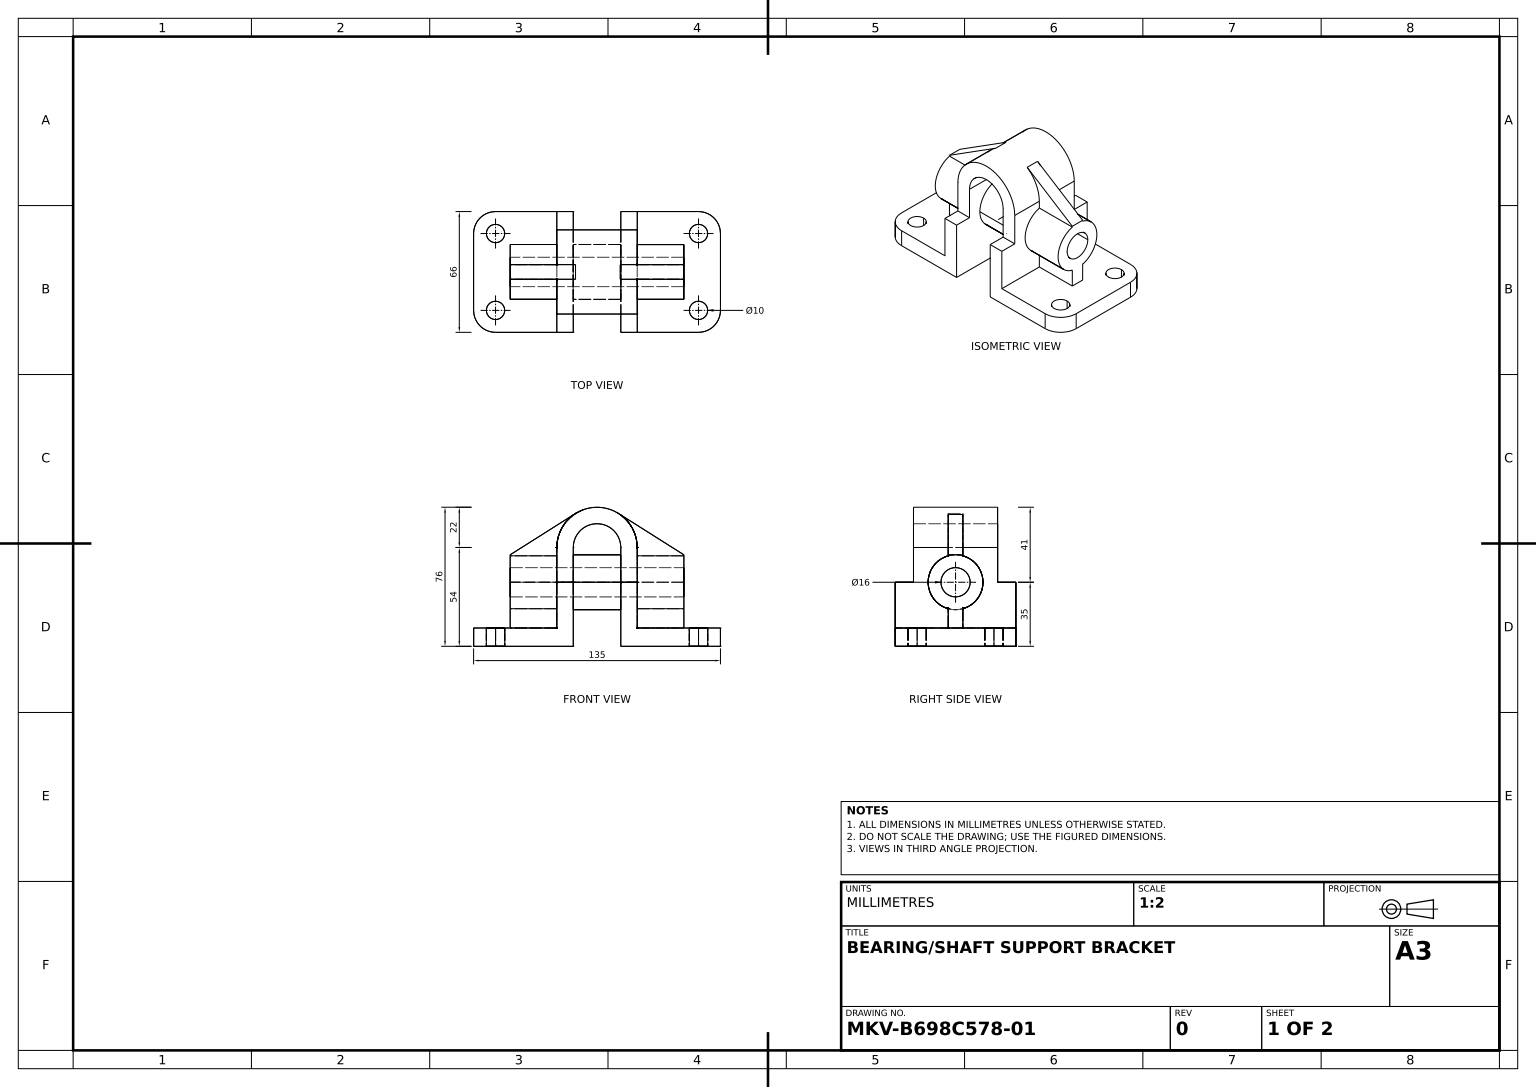
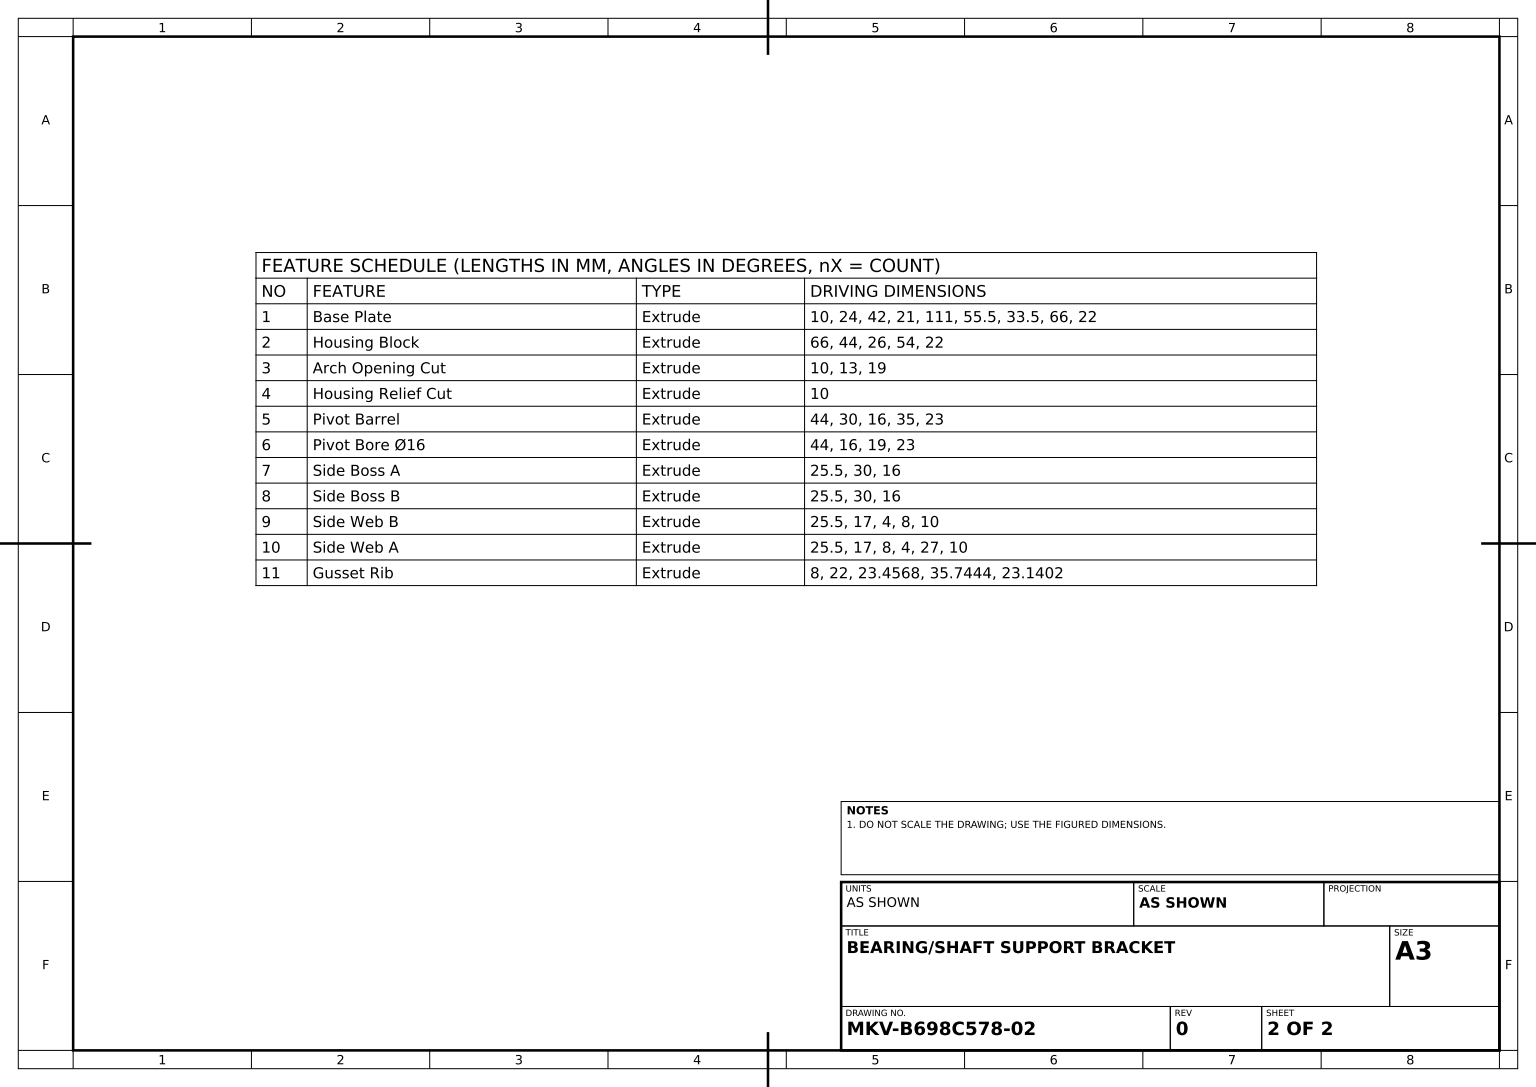
solid
v1 (13,35,15)
v2 (-13,35,15)
e1 v1 v2 LINE
v3 (-13,35,-15)
e2 v2 v3 CIRCLE(AX(P(-13,35,0),D(1,0,0),D(0,0,-1)),15)
v4 (13,35,-15)
e3 v4 v3 LINE
e4 v4 v1 CIRCLE(AX(P(13,35,0),D(-1,0,0),D(0,0,1)),15)
face CYL(AX(P(22,35,0),D(-1,0,0),D(0,0,1)),15) [e1 e2 -e3 e4]
v5 (-67.5,10,21)
v6 (-55.5,10,33)
e5 v5 v6 CIRCLE(AX(P(-55.5,10,21),D(0,1,0),D(0,0,1)),12)
v7 (-67.5,0,21)
e6 v5 v7 LINE
v8 (-55.5,0,33)
e7 v7 v8 CIRCLE(AX(P(-55.5,0,21),D(0,1,0),D(0,0,1)),12)
e8 v6 v8 LINE
face CYL(AX(P(-55.5,10,21),D(0,-1,0),D(0,0,-1)),12) [-e5 e6 e7 -e8]
v9 (-55.5,0,-16)
v10 (-55.5,0,-26)
e9 v9 v10 CIRCLE(AX(P(-55.5,0,-21),D(0,1,0),D(0,0,1)),5)
v11 (-55.5,10,-16)
e10 v11 v9 LINE
v12 (-55.5,10,-26)
e11 v11 v12 CIRCLE(AX(P(-55.5,10,-21),D(0,1,0),D(0,0,1)),5)
e12 v12 v10 LINE
face CYL(AX(P(-55.5,10,-21),D(0,-1,0),D(0,0,-1)),5) rev [-e9 -e10 e11 e12]
v13 (-55.5,10,16)
v14 (-55.5,0,16)
e13 v13 v14 LINE
v15 (-55.5,0,26)
e14 v15 v14 CIRCLE(AX(P(-55.5,0,21),D(0,1,0),D(0,0,1)),5)
v16 (-55.5,10,26)
e15 v16 v15 LINE
e16 v16 v13 CIRCLE(AX(P(-55.5,10,21),D(0,1,0),D(0,0,1)),5)
face CYL(AX(P(-55.5,10,21),D(0,-1,0),D(0,0,-1)),5) rev [e13 -e14 -e15 e16]
v17 (12.61567,72.023453,4)
v18 (22,54,4)
e17 v17 v18 CIRCLE(AX(P(0,54,4),D(0,0,-1),D(1,0,0)),22)
v19 (22,49.456832,4)
e18 v18 v19 LINE
v20 (47.5,49.456832,4)
e19 v20 v19 LINE
v21 (47.5,50,4)
e20 v20 v21 LINE
e21 v21 v17 LINE
face PLANE(AX(P(0,0,4),D(0,0,1),D(1,0,0))) [e17 e18 -e19 e20 e21]
v22 (-22,54,4)
v23 (-22,54,23)
e22 v22 v23 LINE
v24 (-22,49.456832,4)
e23 v24 v22 LINE
v25 (-22,20.543168,4)
e24 v25 v24 CIRCLE(AX(P(-22,35,0),D(-1,0,0),D(0,0,1)),15)
v26 (-22,10,4)
e25 v26 v25 LINE
v27 (-22,10,33)
e26 v27 v26 LINE
v28 (-22,35,33)
e27 v28 v27 LINE
v29 (-22,35,23)
e28 v29 v28 LINE
e29 v23 v29 LINE
face PLANE(AX(P(-22,10,-33),D(-1,0,0),D(0,0,1))) [-e22 -e23 -e24 -e25 -e26 -e27 -e28 -e29]
v30 (-22,49.456832,-4)
v31 (-47.5,49.456832,-4)
e30 v30 v31 LINE
v32 (-22,35,-15)
e31 v30 v32 CIRCLE(AX(P(-22,35,0),D(-1,0,0),D(0,0,1)),15)
v33 (-47.5,35,-15)
e32 v33 v32 LINE
e33 v31 v33 CIRCLE(AX(P(-47.5,35,0),D(-1,0,0),D(0,0,1)),15)
face CYL(AX(P(-47.5,35,0),D(1,0,0),D(0,0,-1)),15) [-e30 e31 -e32 -e33]
v34 (-47.5,10,4)
e34 v26 v34 LINE
v35 (-47.5,20.543168,4)
e35 v35 v25 LINE
e36 v34 v35 LINE
face PLANE(AX(P(-22,27,4),D(0,0,1),D(1,0,0))) [-e34 e25 -e35 -e36]
v36 (67.5,10,21)
v37 (67.5,0,21)
e37 v36 v37 LINE
v38 (55.5,10,33)
e38 v38 v36 CIRCLE(AX(P(55.5,10,21),D(0,1,0),D(0,0,1)),12)
v39 (55.5,0,33)
e39 v38 v39 LINE
e40 v39 v37 CIRCLE(AX(P(55.5,0,21),D(0,1,0),D(0,0,1)),12)
face CYL(AX(P(55.5,10,21),D(0,-1,0),D(0,0,-1)),12) [-e37 -e38 e39 e40]
v40 (47.5,20.543168,-4)
v41 (47.5,10,-4)
e41 v40 v41 LINE
v42 (22,10,-4)
e42 v42 v41 LINE
v43 (22,20.543168,-4)
e43 v43 v42 LINE
e44 v43 v40 LINE
face PLANE(AX(P(22,0,-4),D(0,0,1),D(1,0,0))) rev [e41 -e42 -e43 e44]
v44 (55.5,0,-16)
v45 (55.5,0,-26)
e45 v44 v45 CIRCLE(AX(P(55.5,0,-21),D(0,1,0),D(0,0,1)),5)
v46 (55.5,10,-16)
e46 v46 v44 LINE
v47 (55.5,10,-26)
e47 v46 v47 CIRCLE(AX(P(55.5,10,-21),D(0,1,0),D(0,0,1)),5)
e48 v47 v45 LINE
face CYL(AX(P(55.5,10,-21),D(0,-1,0),D(0,0,-1)),5) rev [-e45 -e46 e47 e48]
e49 v10 v9 CIRCLE(AX(P(-55.5,0,-21),D(0,1,0),D(0,0,1)),5)
e50 v12 v11 CIRCLE(AX(P(-55.5,10,-21),D(0,1,0),D(0,0,1)),5)
face CYL(AX(P(-55.5,10,-21),D(0,-1,0),D(0,0,-1)),5) rev [e10 -e49 -e12 e50]
v48 (13,35,-23)
v49 (13,54,-23)
e51 v48 v49 LINE
v50 (13,35,-33)
e52 v48 v50 LINE
v51 (13,0,-33)
e53 v50 v51 LINE
v52 (13,0,33)
e54 v51 v52 LINE
v53 (13,35,33)
e55 v53 v52 LINE
v54 (13,35,23)
e56 v54 v53 LINE
v55 (13,54,23)
e57 v55 v54 LINE
e58 v49 v55 LINE
e59 v1 v4 CIRCLE(AX(P(13,35,0),D(-1,0,0),D(0,0,1)),15)
face PLANE(AX(P(13,54,-33),D(-1,0,0),D(0,0,1))) [-e51 e52 e53 e54 -e55 -e56 -e57 -e58] [-e4 -e59]
v56 (-47.5,35,8)
v57 (-47.5,35,-8)
e60 v56 v57 CIRCLE(AX(P(-47.5,35,0),D(-1,0,0),D(0,0,1)),8)
v58 (47.5,35,-8)
e61 v58 v57 LINE
v59 (47.5,35,8)
e62 v58 v59 CIRCLE(AX(P(47.5,35,0),D(1,0,0),D(0,1,0)),8)
e63 v59 v56 LINE
face CYL(AX(P(22,35,0),D(-1,0,0),D(0,0,1)),8) rev [e60 -e61 e62 e63]
v60 (-22,35,-23)
v61 (-22,54,-23)
e64 v60 v61 LINE
v62 (-22,35,-33)
e65 v60 v62 LINE
v63 (-22,10,-33)
e66 v62 v63 LINE
v64 (-22,10,-4)
e67 v64 v63 LINE
v65 (-22,20.543168,-4)
e68 v65 v64 LINE
e69 v32 v65 CIRCLE(AX(P(-22,35,0),D(-1,0,0),D(0,0,1)),15)
v66 (-22,54,-4)
e70 v30 v66 LINE
e71 v61 v66 LINE
face PLANE(AX(P(-22,10,-33),D(-1,0,0),D(0,0,1))) [-e64 e65 e66 -e67 -e68 -e69 -e31 e70 -e71]
e72 v14 v15 CIRCLE(AX(P(-55.5,0,21),D(0,1,0),D(0,0,1)),5)
v67 (-55.5,0,-33)
v68 (-13,0,-33)
e73 v67 v68 LINE
v69 (-13,0,33)
e74 v68 v69 LINE
e75 v8 v69 LINE
v70 (-67.5,0,-21)
e76 v70 v7 LINE
e77 v67 v70 CIRCLE(AX(P(-55.5,0,-21),D(0,1,0),D(0,0,1)),12)
face PLANE(AX(P(-22,0,-33),D(0,-1,0),D(0,0,-1))) [e72 e14] [e49 e9] [e73 e74 -e75 -e7 -e76 -e77]
v71 (-47.5,50,-4)
v72 (-11.755648,72.595826,-4)
e78 v71 v72 LINE
e79 v66 v72 CIRCLE(AX(P(0,54,-4),D(0,0,-1),D(1,0,0)),22)
e80 v71 v31 LINE
face PLANE(AX(P(0,0,-4),D(0,0,1),D(1,0,0))) rev [e78 -e79 -e70 e30 -e80]
v73 (47.5,20.543168,4)
e81 v20 v73 CIRCLE(AX(P(47.5,35,0),D(1,0,0),D(0,1,0)),15)
v74 (47.5,10,4)
e82 v73 v74 LINE
e83 v41 v74 LINE
v75 (47.5,49.456832,-4)
e84 v40 v75 CIRCLE(AX(P(47.5,35,0),D(1,0,0),D(0,1,0)),15)
v76 (47.5,50,-4)
e85 v75 v76 LINE
e86 v21 v76 LINE
e87 v59 v58 CIRCLE(AX(P(47.5,35,0),D(1,0,0),D(0,1,0)),8)
face PLANE(AX(P(47.5,35,0),D(1,0,0),D(0,1,0))) [-e20 e81 e82 -e83 -e41 e84 e85 -e86] [-e87 -e62]
v77 (22,35,23)
v78 (22,35,33)
e88 v77 v78 LINE
e89 v54 v77 LINE
e90 v53 v78 LINE
face PLANE(AX(P(0,35,23),D(0,-1,0),D(0,0,-1))) rev [-e88 -e89 e56 e90]
v79 (-13,35,-33)
e91 v79 v62 LINE
v80 (-13,35,-23)
e92 v80 v60 LINE
e93 v80 v79 LINE
face PLANE(AX(P(-13,35,-23),D(0,-1,0),D(0,0,-1))) rev [e91 -e65 -e92 e93]
v81 (67.5,0,-21)
e94 v37 v81 LINE
v82 (67.5,10,-21)
e95 v82 v81 LINE
e96 v36 v82 LINE
face PLANE(AX(P(67.5,10,-21),D(-1,0,0),D(0,0,1))) rev [e37 e94 -e95 -e96]
v83 (-47.5,20.543168,-4)
v84 (-47.5,10,-4)
e97 v83 v84 LINE
e98 v65 v83 LINE
e99 v64 v84 LINE
face PLANE(AX(P(-22,27,-4),D(0,0,-1),D(-1,0,0))) [-e97 -e98 e68 e99]
v85 (55.5,0,-33)
e100 v85 v51 LINE
v86 (22,35,-33)
e101 v86 v50 LINE
v87 (22,10,-33)
e102 v87 v86 LINE
v88 (55.5,10,-33)
e103 v88 v87 LINE
e104 v88 v85 LINE
face PLANE(AX(P(55.5,10,-33),D(0,0,1),D(1,0,0))) rev [e100 -e53 -e101 -e102 -e103 e104]
v89 (-13,35,33)
e105 v89 v28 LINE
v90 (-13,35,23)
e106 v90 v89 LINE
e107 v90 v29 LINE
face PLANE(AX(P(0,35,23),D(0,1,0),D(0,0,1))) [-e105 -e106 e107 e28]
v91 (55.5,0,26)
v92 (55.5,0,16)
e108 v91 v92 CIRCLE(AX(P(55.5,0,21),D(0,1,0),D(0,0,1)),5)
v93 (55.5,10,26)
e109 v93 v91 LINE
v94 (55.5,10,16)
e110 v93 v94 CIRCLE(AX(P(55.5,10,21),D(0,1,0),D(0,0,1)),5)
e111 v94 v92 LINE
face CYL(AX(P(55.5,10,21),D(0,-1,0),D(0,0,-1)),5) rev [-e108 -e109 e110 e111]
v95 (12.61567,72.023453,-4)
e112 v76 v95 LINE
e113 v17 v95 LINE
face PLANE(AX(P(36.10726,57.192555,4),D(-0.533841277,-0.845584704,0),D(0.845584704,-0.533841277,0))) rev [-e21 e86 e112 -e113]
e114 v47 v46 CIRCLE(AX(P(55.5,10,-21),D(0,1,0),D(0,0,1)),5)
e115 v45 v44 CIRCLE(AX(P(55.5,0,-21),D(0,1,0),D(0,0,1)),5)
face CYL(AX(P(55.5,10,-21),D(0,-1,0),D(0,0,-1)),5) rev [-e48 e114 e46 -e115]
v96 (-47.5,49.456832,4)
e116 v35 v96 CIRCLE(AX(P(-47.5,35,0),D(-1,0,0),D(0,0,1)),15)
v97 (-47.5,50,4)
e117 v97 v96 LINE
e118 v97 v71 LINE
e119 v33 v83 CIRCLE(AX(P(-47.5,35,0),D(-1,0,0),D(0,0,1)),15)
e120 v84 v34 LINE
e121 v57 v56 CIRCLE(AX(P(-47.5,35,0),D(-1,0,0),D(0,0,1)),8)
face PLANE(AX(P(-47.5,35,0),D(-1,0,0),D(0,0,1))) [e116 -e117 e118 e80 e33 e119 e97 e120 e36] [-e60 -e121]
v98 (22,49.456832,-4)
e122 v75 v98 LINE
v99 (22,54,-4)
e123 v99 v98 LINE
e124 v95 v99 CIRCLE(AX(P(0,54,-4),D(0,0,-1),D(1,0,0)),22)
face PLANE(AX(P(0,0,-4),D(0,0,1),D(1,0,0))) rev [-e112 -e85 e122 -e123 -e124]
v100 (-67.5,10,-21)
e125 v100 v5 LINE
e126 v100 v70 LINE
face PLANE(AX(P(-67.5,10,-21),D(1,0,0),D(0,0,-1))) rev [-e6 -e125 e126 e76]
e127 v81 v85 CIRCLE(AX(P(55.5,0,-21),D(0,1,0),D(0,0,1)),12)
e128 v52 v39 LINE
e129 v92 v91 CIRCLE(AX(P(55.5,0,21),D(0,1,0),D(0,0,1)),5)
face PLANE(AX(P(55.5,0,-21),D(0,1,0),D(0,0,1))) rev [e45 e115] [-e127 -e94 -e40 -e128 -e54 -e100] [e129 e108]
e130 v6 v27 LINE
e131 v69 v89 LINE
face PLANE(AX(P(22,10,33),D(0,0,-1),D(-1,0,0))) rev [e105 e27 -e130 e8 e75 e131]
e132 v94 v93 CIRCLE(AX(P(55.5,10,21),D(0,1,0),D(0,0,1)),5)
e133 v82 v88 CIRCLE(AX(P(55.5,10,-21),D(0,1,0),D(0,0,1)),12)
e134 v87 v42 LINE
v101 (22,10,4)
e135 v101 v74 LINE
v102 (22,10,33)
e136 v101 v102 LINE
e137 v102 v38 LINE
face PLANE(AX(P(55.5,10,-21),D(0,1,0),D(0,0,1))) [-e110 -e132] [-e114 -e47] [e96 e133 e103 e134 e42 e83 -e135 e136 e137 e38]
e138 v3 v2 CIRCLE(AX(P(-13,35,0),D(1,0,0),D(0,0,-1)),15)
face CYL(AX(P(22,35,0),D(-1,0,0),D(0,0,1)),15) [e59 e3 e138 -e1]
v103 (-13,54,-23)
e139 v49 v103 CIRCLE(AX(P(0,54,-23),D(0,0,1),D(1,0,0)),13)
v104 (-13,54,23)
e140 v104 v55 CIRCLE(AX(P(0,54,23),D(0,0,-1),D(1,0,0)),13)
e141 v103 v104 LINE
face CYL(AX(P(0,54,-33),D(0,0,1),D(1,0,0)),13) rev [-e139 e58 -e140 -e141]
e142 v24 v96 LINE
v105 (-11.755648,72.595826,4)
e143 v22 v105 CIRCLE(AX(P(0,54,4),D(0,0,-1),D(1,0,0)),22)
e144 v97 v105 LINE
face PLANE(AX(P(0,0,4),D(0,0,1),D(1,0,0))) [-e142 e23 e143 -e144 e117]
e145 v43 v98 CIRCLE(AX(P(22,35,0),D(1,0,0),D(0,1,0)),15)
face CYL(AX(P(47.5,35,0),D(-1,0,0),D(0,-1,0)),15) [-e84 -e44 e145 -e122]
face CYL(AX(P(55.5,10,-21),D(0,-1,0),D(0,0,-1)),12) [-e133 e95 e127 -e104]
v106 (22,35,-23)
e146 v106 v86 LINE
v107 (22,54,-23)
e147 v107 v106 LINE
e148 v107 v99 LINE
face PLANE(AX(P(22,0,-33),D(1,0,0),D(0,1,0))) [e123 -e145 e43 -e134 e102 -e146 -e147 e148]
face CYL(AX(P(-47.5,35,0),D(1,0,0),D(0,0,-1)),15) [e35 e24 e142 -e116]
v108 (22,20.543168,4)
e149 v108 v73 LINE
e150 v108 v101 LINE
face PLANE(AX(P(22,0,4),D(0,0,1),D(1,0,0))) [-e82 -e149 e150 e135]
v109 (22,54,23)
e151 v77 v109 LINE
e152 v109 v23 CIRCLE(AX(P(0,54,23),D(0,0,1),D(1,0,0)),22)
e153 v90 v104 LINE
face PLANE(AX(P(0,0,23),D(0,0,1),D(1,0,0))) [e57 e89 e151 e152 e29 -e107 e153 e140]
v110 (-55.5,10,-33)
e154 v110 v100 CIRCLE(AX(P(-55.5,10,-21),D(0,1,0),D(0,0,1)),12)
e155 v110 v67 LINE
face CYL(AX(P(-55.5,10,-21),D(0,-1,0),D(0,0,-1)),12) [-e126 -e154 e155 e77]
e156 v102 v78 LINE
face PLANE(AX(P(22,10,33),D(0,0,-1),D(-1,0,0))) rev [e156 -e90 e55 e128 -e39 -e137]
e157 v106 v48 LINE
face PLANE(AX(P(13,35,-23),D(0,-1,0),D(0,0,-1))) rev [-e157 e146 e101 -e52]
e158 v63 v110 LINE
e159 v13 v16 CIRCLE(AX(P(-55.5,10,21),D(0,1,0),D(0,0,1)),5)
face PLANE(AX(P(-55.5,10,-21),D(0,1,0),D(0,0,1))) [e34 -e120 -e99 e67 e158 e154 e125 e5 e130 e26] [-e50 -e11] [-e159 -e16]
e160 v61 v107 CIRCLE(AX(P(0,54,-23),D(0,0,-1),D(1,0,0)),22)
e161 v105 v72 LINE
e162 v18 v109 LINE
face CYL(AX(P(0,54,-33),D(0,0,1),D(1,0,0)),22) [e113 e124 -e148 -e160 e71 e79 -e161 -e143 e22 -e152 -e162 -e17]
e163 v103 v80 LINE
face PLANE(AX(P(0,54,-23),D(0,0,1),D(1,0,0))) rev [e147 e157 e51 e139 e163 e92 e64 e160]
face CYL(AX(P(22,35,0),D(-1,0,0),D(0,0,1)),8) rev [e61 e121 -e63 e87]
face CYL(AX(P(-55.5,10,21),D(0,-1,0),D(0,0,-1)),5) rev [-e72 -e13 e159 e15]
e164 v19 v108 CIRCLE(AX(P(22,35,0),D(1,0,0),D(0,1,0)),15)
face PLANE(AX(P(22,0,-33),D(1,0,0),D(0,1,0))) [-e151 e88 -e156 -e136 -e150 -e164 -e18 e162]
face CYL(AX(P(-47.5,35,0),D(1,0,0),D(0,0,-1)),15) [e98 -e119 e32 e69]
e165 v68 v79 LINE
face PLANE(AX(P(-13,0,-33),D(1,0,0),D(0,0,-1))) [-e138 -e2] [-e74 e165 -e93 -e163 e141 -e153 e106 -e131]
face PLANE(AX(P(-36.145124,57.177996,4),D(-0.534338572,0.845270543,0),D(-0.845270543,-0.534338572,0))) [-e78 -e118 e144 e161]
face CYL(AX(P(55.5,10,21),D(0,-1,0),D(0,0,-1)),5) rev [-e111 e132 e109 -e129]
face PLANE(AX(P(55.5,10,-33),D(0,0,1),D(1,0,0))) rev [-e66 -e91 -e165 -e73 -e155 -e158]
face CYL(AX(P(47.5,35,0),D(-1,0,0),D(0,-1,0)),15) [-e81 e19 e164 e149]
